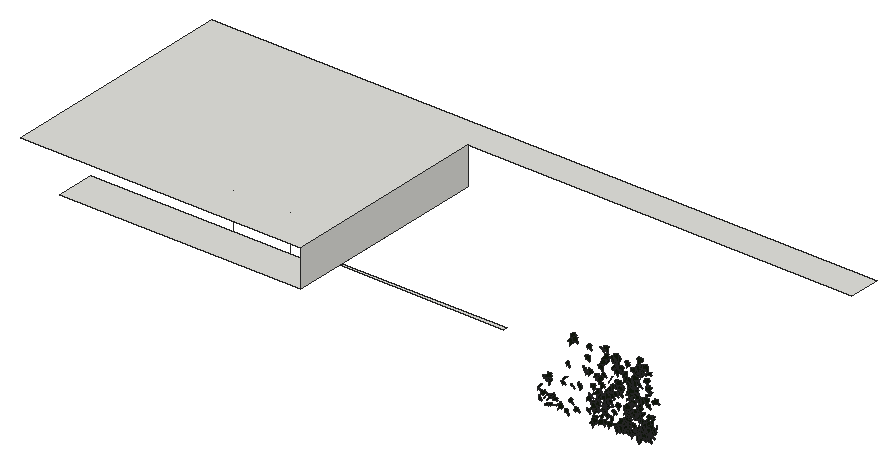
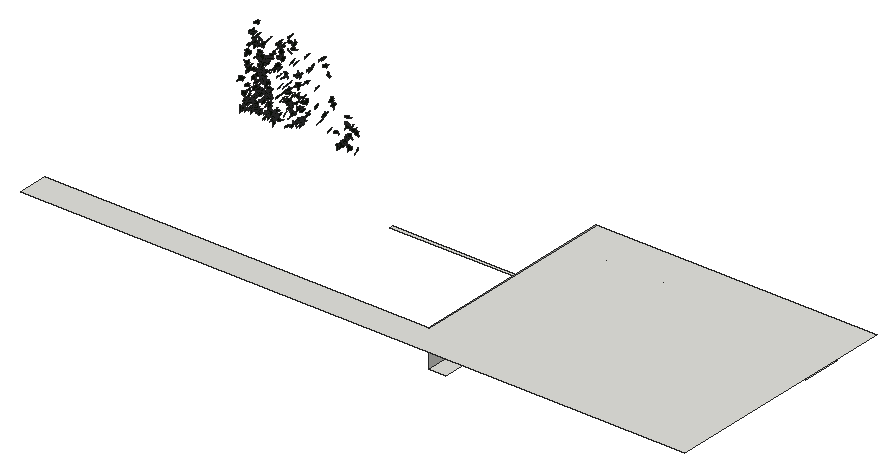
# SketchUp Ruby script. Lengths in inches.
U = 1.inch
M = Sketchup.active_model
def pt(a) = Geom::Point3d.new(a.map { |v| v * U })
def face(e, loops, mat)
  f = e.add_face(loops[0].map { |a| pt(a) })
  loops[1..].each { |l| e.add_face(l.map { |a| pt(a) }).erase! }
  f.material = f.back_material = mat if mat
  f
end
# faces: each face lists its corners as indices into pts; further lists are holes
def faces(e, pts, list, mat = nil) = list.each { |f| face(e, (f[0].is_a?(Array) ? f : [f]).map { |l| l.map { |i| pts[i] } }, mat) }
# xy, xz, yz: faces in a plane at the given z, y or x. An outline is a flat list of corners, or four numbers for a rectangle; further outlines are holes
def ring(l) = l.size == 4 ? [[l[0], l[1]], [l[2], l[1]], [l[2], l[3]], [l[0], l[3]]] : l.each_slice(2).to_a
def flat(e, list, mat, &to3) = list.each { |f| face(e, (f[0].is_a?(Array) ? f : [f]).map { |l| ring(l).map { |u, v| to3.(u, v) } }, mat) }
def xy(e, z, list, mat = nil) = flat(e, list, mat) { |x, y| [x, y, z] }
def xz(e, y, list, mat = nil) = flat(e, list, mat) { |x, z| [x, y, z] }
def yz(e, x, list, mat = nil) = flat(e, list, mat) { |y, z| [x, y, z] }
def lines(e, pts, list) = list.each { |a, b| e.add_line(pt(pts[a]), pt(pts[b])) }
# prism: a flat outline (further loops are holes) pulled along v
def prism(e, loops, v, mat = nil)
  f = face(e, loops, mat); d = Geom::Vector3d.new(v.map { |x| x * U })
  f.pushpull(f.normal.samedirection?(d) ? d.length : -d.length)
end
def box(e, o, s, mat = nil) = prism(e, [[o, [o[0] + s[0], o[1], o[2]], [o[0] + s[0], o[1] + s[1], o[2]], [o[0], o[1] + s[1], o[2]]]], [0, 0, s[2]], mat)
def at(x, y, z, deg = 0) = Geom::Transformation.translation(pt([x, y, z])) * Geom::Transformation.rotation(ORIGIN, Z_AXIS, deg.degrees)
def axes(o, x, y, z) = Geom::Transformation.new([*x, 0, *y, 0, *z, 0, *pt(o).to_a, 1])
def part(name) = M.definitions.add(name)
# library, detail: a bought-in or finely detailed component or shape, given as its bounding box
def library(name, o, s) = part(name).tap { |d| box(d.entities, o, s) }
def detail(e, o, s) = box(e.add_group.entities, o, s)
def put(e, d, t, mat = nil) = e.add_instance(d, t).tap { |i| i.material = mat if mat }
def group(e, t, mat = nil) = e.add_group.tap { |g| g.transformation = t; g.material = mat if mat }.entities
root = M.entities
M.materials.add("efeu1").color = [18, 25, 13]
c1 = part("ivyleaf_9")
p = [[1.54,2.16,1.25],[1.36,2.04,1.19],[-0.21,0.99,0.68],[-0.71,1.11,0.82],[-0.85,0.86,0.67],[-0.8,0.17,0.21],
  [-0.9,-0.01,0.1],[-0.67,-0.16,-0.02],[-0.08,-0.08,-0.05],[-0.03,-0.6,-0.4],[0.65,-0.88,-0.66],[0.83,-0.6,-0.49],
  [1.29,-0.42,-0.43],[1.8125,-0.07,-0.26],[1.21,0.44,0.15]]
faces(c1.entities,p,[[0,1,2,3,4,5,6,7,8,9,10,11,12,13,14]],"efeu1")
xy(root,328.1875,[[63.85,139.625,270.19,172.6875],[255.63,172.6875,270.19,181.4375],[270.19,181.4375,411.76,184.12],[255.63,184.12,270.19,319]])
xy(root,360,[[29.66,139.625,270.19,139.625,270.19,319,600,319,600,345.4375,29.66,345.4375]])
yz(root,270.19,[[139.625,328.1875,319,360]])
p = [[186.23,172.6875,360],[186.23,172.6875,328.1875],[235.22,172.6875,360],[235.22,172.6875,328.1875]]
lines(root,p,[[0,1],[2,3]])
put(root,c1,axes([491.06,119.55,331.81],[0.98321,-0.43675,-0.79022],[-0.6769,0.44134,-1.04482],[0.6616,1.10061,0.10539]))
put(root,c1,axes([494.23,116.77,342.93],[-0.50471,0.9603,-0.79093],[0.29874,-0.71022,-1.10944],[-1.2888,-0.54069,0.05257]))
put(root,c1,axes([494.78,120.51,348.57],[0.8379,-1.02369,-0.06234],[-0.00036,0.07491,-1.33503],[1.10748,0.77453,0.04673]))
put(root,c1,axes([499.15,117.69,329.99],[0.74075,1.01696,0.13512],[0.07482,0.10999,-1.2757],[-1.10472,0.68936,0.00421]))
put(root,c1,axes([499.41,119.17,347.66],[0.9407,0.95541,0.26934],[-0.05629,0.38876,-1.3092],[-1.06759,0.82135,0.30636]))
put(root,c1,axes([500.5,113.04,340.41],[0.17657,0.26151,1.32901],[-1.3928,0.22553,0.1236],[-0.21124,-1.26842,0.29598]))
put(root,c1,axes([500.88,120.67,335.94],[-0.15345,1.13375,-0.52577],[-0.03576,-0.51213,-1.18477],[-1.34019,-0.11615,0.09182]))
put(root,c1,axes([501.08,116.4375,338.25],[-0.68537,0.89054,-0.64163],[0.04243,-0.69561,-1.08628],[-1.16927,-0.54723,0.33667]))
put(root,c1,axes([500.22,119.6875,348.3],[-0.81391,-0.69586,-0.81701],[0.86609,0.24203,-1.02303],[0.73112,-1.06137,0.30237]))
put(root,c1,axes([501.71,121.67,334.63],[-0.43261,0.2825,1.18213],[-1.00858,0.648,-0.50976],[-0.76344,-1.01615,0.00357]))
put(root,c1,axes([500.99,119.21,348.96],[-1.09001,-0.37422,-0.73907],[0.73045,0.21948,-1.11918],[0.46779,-1.21469,0.02546]))
put(root,c1,axes([502.0625,118.14,352.8],[-1.15304,-0.11068,0.76991],[-0.75428,-0.31667,-1.09673],[0.29085,-1.26,0.20801]))
put(root,c1,axes([502.59,115.34,335.8],[0.51297,0.78721,0.95609],[0.19946,0.92887,-0.92644],[-1.29182,0.45601,0.23661]))
put(root,c1,axes([502.41,122.02,332.98],[0.89619,0.87408,0.14744],[0.1088,0.09984,-1.25343],[-0.95013,0.83588,-0.00446]))
put(root,c1,axes([504.23,114.77,332.87],[1.11009,0.20793,0.82745],[0.82025,0.24831,-1.08792],[-0.34055,1.27588,0.07688]))
put(root,c1,axes([506.18,121.38,330.43],[0.12532,1.05764,0.69606],[-0.04469,0.67503,-1.10193],[-1.35101,0.07578,0.10101]))
put(root,c1,axes([514.375,114.71,335.34],[-1.21116,-0.52096,0.19612],[-0.1902,-0.05406,-1.31821],[0.52315,-1.22574,-0.02521]))
put(root,c1,axes([517.23,112.87,355.13],[0.79088,0.38712,-1.07511],[-1.00802,-0.37942,-0.87815],[-0.53815,1.2796,0.06487]))
put(root,c1,axes([517.92,112.67,357.73],[0.58616,0.65304,1.08802],[0.47943,0.99569,-0.85591],[-1.1749,0.7321,0.19356]))
put(root,c1,axes([517.82,120.96,349.81],[1.09478,-0.78677,0.26516],[0.2539,-0.10053,-1.34658],[0.79047,1.12194,0.06528]))
put(root,c1,axes([519.67,112.89,334.43],[0.65078,-1.15916,-0.29844],[-0.0944,0.28894,-1.32809],[1.19324,0.65505,0.05769]))
put(root,c1,axes([520.5,118.41,385.79],[-0.91086,-1.13881,0.03125],[-0.02038,-0.02372,-1.45827],[1.13906,-0.91109,-0.0011]))
put(root,c1,axes([521.77,118.1,391.04],[0.04989,-1.401,-0.45119],[0.17121,0.45391,-1.3905],[1.46187,-0.00535,0.17825]))
put(root,c1,axes([523.41,117.5,389.22],[0.1852,-1.18685,-0.84705],[0.38674,0.86326,-1.125],[1.4059,-0.08112,0.42105]))
put(root,c1,axes([523.42,109.72,373.73],[-0.03799,-0.29316,-1.43905],[1.43722,0.2886,-0.09674],[0.302,-1.41032,0.27934]))
put(root,c1,axes([524.04,112.02,344.46],[0.76113,-1.06438,-0.49172],[-0.16172,0.48534,-1.30088],[1.16126,0.76522,0.14113]))
put(root,c1,axes([525.49,120.44,353.23],[0.724,-1.03353,0.55169],[0.2756,-0.48009,-1.26106],[1.13868,0.77334,-0.04555]))
put(root,c1,axes([527.59,113.15,338.16],[0.80232,-0.79111,-0.80628],[-0.19572,0.87665,-1.05491],[1.11249,0.72477,0.39589]))
put(root,c1,axes([532.34,121.27,344.83],[0.40368,-1.09674,-0.68829],[-0.07448,0.7001,-1.15924],[1.29269,0.38282,0.14815]))
put(root,c1,axes([533.79,118.08,378.62],[0.54183,-1.18623,-0.64307],[-0.12496,0.64589,-1.29672],[1.34353,0.53846,0.13873]))
put(root,c1,axes([533.74,110.12,359.84],[0.25984,-1.28174,0.64002],[0.22372,-0.60618,-1.3048],[1.41507,0.3312,0.08876]))
put(root,c1,axes([535.62,119.13,368.05],[-0.55222,-1.3096,0.07111],[-0.01992,-0.06877,-1.42124],[1.31138,-0.55252,0.00835]))
put(root,c1,axes([535.74,117.19,387.75],[0.61048,-1.22558,-0.56432],[-0.00111,0.61894,-1.3454],[1.34926,0.55503,0.25422]))
put(root,c1,axes([535.8,121.87,337.8125],[0.39608,-0.95937,0.84674],[0.3218,-0.78321,-1.03792],[1.23847,0.51033,-0.00111]))
put(root,c1,axes([537.04,120.18,356.61],[0.00922,-1.33902,-0.38342],[0.01688,0.38351,-1.33892],[1.39273,0.00421,0.01877]))
put(root,c1,axes([536.73,116.47,351.33],[1.29715,-0.55053,0.23449],[0.21062,-0.1039,-1.40908],[0.56009,1.31407,-0.01317]))
put(root,c1,axes([537.36,109.94,375.16],[1.0725,-1.04548,-0.03075],[-0.0239,0.01953,-1.49776],[1.04566,1.07276,-0.0027]))
put(root,c1,axes([537.8125,114.01,340.61],[0.57296,-1.14178,0.59781],[0.41423,-0.45636,-1.26865],[1.22043,0.69093,0.14994]))
put(root,c1,axes([539.49,121.83,339.83],[-1.34684,-0.00456,0.09388],[-0.09385,-0.00694,-1.34683],[0.00503,-1.35009,0.00661]))
put(root,c1,axes([538.35,111.18,371.94],[0.12554,-1.21301,0.85578],[0.26277,-0.82712,-1.21092],[1.46106,0.25298,0.14425]))
put(root,c1,axes([539.84,121.57,338.15],[-0.73475,-1.00394,0.51386],[-0.30506,-0.41352,-1.24409],[1.08577,-0.79557,-0.00181]))
put(root,c1,axes([539.1,121.5625,339.9],[0.3193,-1.07225,-0.76696],[0.15763,0.81452,-1.07313],[1.30886,0.16349,0.31634]))
put(root,c1,axes([539.65,118.93,344.67],[-0.49458,-1.26783,0.04544],[-0.00699,-0.04605,-1.36085],[1.26863,-0.49452,0.01022]))
put(root,c1,axes([539.65,119.3,333.49],[-0.08067,-1.21087,-0.54346],[0.20773,0.52624,-1.20332],[1.31088,-0.15791,0.15725]))
put(root,c1,axes([540.33,120.63,346.7],[0.42987,-0.73139,-1.07949],[-0.23869,1.0733,-0.82225],[1.2819,0.44511,0.20889]))
put(root,c1,axes([542.24,119.26,364.2],[0.06702,1.41664,-0.05834],[-0.00082,-0.05837,-1.41823],[-1.41784,0.067,-0.00194]))
put(root,c1,axes([543.33,118.47,344.83],[-0.73484,-0.28673,1.11502],[-0.96495,-0.56812,-0.78203],[0.62797,-1.20851,0.10308]))
put(root,c1,axes([542.84,113.71,333.02],[-0.56445,-1.32849,-0.20518],[0.09095,0.18428,-1.44338],[1.34116,-0.57162,0.01152]))
put(root,c1,axes([542.84,120.52,350.21],[-0.26979,-1.3436,-0.18841],[0.01274,0.18958,-1.3702],[1.35668,-0.26897,-0.0246]))
put(root,c1,axes([544.11,121.46,334.64],[-0.76329,0.95569,0.57248],[-0.37002,0.43708,-1.223],[-1.05079,-0.84812,0.01482]))
put(root,c1,axes([543.71,113.74,335.36],[-0.46046,-1.26984,-0.02353],[-0.0079,0.02789,-1.35064],[1.27003,-0.46022,-0.01693]))
put(root,c1,axes([544.38,112.42,346.89],[-1.06212,-0.92998,0.44622],[-0.30903,-0.32417,-1.4112],[0.98411,-1.1055,0.03845]))
put(root,c1,axes([544.59,118.63,354.44],[-1.30914,-0.45963,-0.17804],[0.16026,0.08089,-1.38729],[0.46612,-1.31872,-0.02305]))
put(root,c1,axes([544.26,115.54,369.02],[-0.09958,-1.46951,-0.22114],[0.12992,0.21218,-1.46846],[1.48037,-0.11747,0.114]))
put(root,c1,axes([544.1875,114.82,366.9],[-0.19262,0.41185,1.41968],[0.62963,-1.27246,0.45457],[1.33742,0.65837,-0.00954]))
put(root,c1,axes([545.0625,116.96,353.93],[-0.21059,-1.3596,0.21791],[-0.06245,-0.21078,-1.3755],[1.37553,-0.21772,-0.02909]))
put(root,c1,axes([546.36,120.9,342.64],[-1.35822,-0.18615,0.01166],[-0.00507,-0.04877,-1.37009],[0.18644,-1.35739,0.04763]))
put(root,c1,axes([545.75,116.85,333],[0.23775,-0.63453,-1.24816],[-0.0975,1.25544,-0.65681],[1.39679,0.19564,0.1666]))
put(root,c1,axes([546.14,119.17,360.43],[-0.48389,-1.23962,0.49954],[-0.01822,-0.5251,-1.32071],[1.33636,-0.45602,0.16287]))
put(root,c1,axes([546.32,120.65,331.78],[-0.02987,-1.31064,-0.22703],[0.04879,0.22586,-1.31027],[1.32926,-0.03774,0.04299]))
put(root,c1,axes([546.4,120.81,341.39],[-0.79827,-0.58379,-0.95076],[0.7634,0.56673,-0.98896],[0.81362,-1.10454,-0.00491]))
put(root,c1,axes([546.9,115.72,368.06],[-0.76626,-1.26593,-0.27277],[0.13242,0.23868,-1.47974],[1.28819,-0.77756,-0.01014]))
put(root,c1,axes([547.66,120.25,346.92],[-0.43565,1.30172,0.21151],[-0.07545,0.19778,-1.37266],[-1.31663,-0.44205,0.00868]))
put(root,c1,axes([546.97,120.5,345.48],[0.41961,-1.30874,0.10938],[0.02131,-0.10802,-1.37431],[1.31313,0.41996,-0.01265]))
put(root,c1,axes([547.01,115.55,377.09],[0.44048,-1.33393,-0.39082],[0.04365,0.42305,-1.39473],[1.38932,0.40963,0.16773]))
put(root,c1,axes([548.52,112.09,359.16],[-1.14594,-0.38162,0.74556],[-0.65746,-0.37291,-1.2014],[0.51889,-1.31529,0.1243]))
put(root,c1,axes([547.4,121.18,337.97],[0.40046,-1.2942,-0.11492],[0.07446,0.14291,-1.35003],[1.29716,0.39135,0.11297]))
put(root,c1,axes([547.74,120.38,347.16],[0.1495,-1.3587,-0.23646],[-0.00123,0.23772,-1.36669],[1.37913,0.1475,0.02441]))
put(root,c1,axes([548.58,120.67,344.11],[-0.53144,-1.22449,-0.33365],[0.10004,0.32018,-1.3344],[1.26519,-0.53966,-0.03464]))
put(root,c1,axes([548.23,117.41,352.58],[0.49896,-1.29655,-0.07612],[-0.01852,0.07443,-1.38921],[1.29865,0.49921,0.00943]))
put(root,c1,axes([548.57,115.51,390.3],[1.28415,-0.54338,-0.53235],[0.49245,-0.20228,1.39438],[-0.57979,-1.37533,0.00525]))
put(root,c1,axes([549.17,120.35,347.43],[-0.18004,-1.37168,0.08],[0.00557,-0.08141,-1.38335],[1.374,-0.1794,0.01609]))
put(root,c1,axes([549.84,122.29,330.59],[-0.41488,-1.24005,0.23911],[0.02109,-0.25846,-1.30375],[1.26272,-0.40311,0.10034]))
put(root,c1,axes([549.92,119.85,355.05],[-0.66417,-1.19263,-0.35048],[0.29432,0.23519,-1.35808],[1.20772,-0.71319,0.13823]))
put(root,c1,axes([550.86,119.23,357.02],[-0.45888,-1.3419,0.0499],[0.00555,-0.05463,-1.41801],[1.34282,-0.45834,0.02291]))
put(root,c1,axes([551.22,117.83,346.42],[0.92221,-0.22884,1.07308],[1.08452,-0.02249,-0.93683],[0.16641,1.41473,0.15868]))
put(root,c1,axes([551.92,119.37,355.77],[0.22405,-1.38648,-0.15003],[0.01643,0.15456,-1.40388],[1.39448,0.22094,0.04064]))
put(root,c1,axes([551.95,120.04,350.02],[0.73144,-1.16552,-0.24444],[-0.00873,0.28161,-1.36887],[1.19085,0.71794,0.14011]))
put(root,c1,axes([553.52,111.91,384.13],[-1.31169,-0.42145,0.57101],[-0.40666,-0.53709,-1.33056],[0.58164,-1.32595,0.35746]))
put(root,c1,axes([552.33,119.125,359.71],[0.7425,-1.04326,-0.62084],[-0.05781,0.69654,-1.2396],[1.21264,0.67199,0.32104]))
put(root,c1,axes([554.07,113.72,382.65],[0.07518,0.77287,1.25945],[-0.69178,1.13276,-0.65383],[-1.30576,-0.55563,0.41891]))
put(root,c1,axes([553.06,110.86,374.84],[1.10105,-0.55116,-0.78981],[-0.50791,0.68695,-1.18744],[0.81829,1.16799,0.32569]))
put(root,c1,axes([554.18,117.99,368.17],[-0.77945,1.18919,-0.29571],[0.1738,-0.23963,-1.4218],[-1.21302,-0.79847,-0.0137]))
put(root,c1,axes([553.37,119.94,337.17],[0.11202,-1.0973,0.79828],[0.07097,-0.79516,-1.10297],[1.35509,0.13236,-0.00822]))
put(root,c1,axes([553.45,119.66,354.84],[0.7894,-1.09313,-0.41091],[-0.01398,0.4871,-1.32267],[1.16773,0.7448,0.26195]))
put(root,c1,axes([553.58,113.3,394.86],[0.32174,-1.42081,-0.39279],[0.04557,0.41144,-1.45091],[1.4734,0.29753,0.13065]))
put(root,c1,axes([554.42,113.71,350.64],[-0.17262,0.80836,1.24038],[0.02741,-1.24682,0.81637],[1.48028,0.11735,0.12953]))
put(root,c1,axes([556.02,111.97,388.9],[-1.45196,-0.00649,0.40098],[-0.401,0.04278,-1.45134],[-0.00514,-1.50571,-0.04296]))
put(root,c1,axes([554.9375,113.98,357.45],[-0.41628,-1.1614,0.84505],[-0.07715,-0.86048,-1.22061],[1.43423,-0.38338,0.17962]))
put(root,c1,axes([556.46,118.52,363.5],[-0.65955,-1.19456,0.45534],[0.00417,-0.51437,-1.3434],[1.27839,-0.61462,0.2393]))
put(root,c1,axes([557.92,121.16,332.03],[-0.68805,0.31455,1.08157],[-1.12576,-0.23406,-0.6481],[0.03734,-1.26033,0.3903]))
put(root,c1,axes([556.49,117.54,377.43],[0.34207,0.23819,1.41732],[0.99117,1.01591,-0.40995],[-1.04073,1.04582,0.07542]))
put(root,c1,axes([557.01,118.91,357.79],[0.85726,-1.00618,-0.51554],[-0.13791,0.54909,-1.30099],[1.12213,0.83617,0.23396]))
put(root,c1,axes([558.49,116.65,383.05],[1.12006,0.3491,-0.93058],[-0.9448,-0.0613,-1.16017],[-0.30856,1.45491,0.17441]))
put(root,c1,axes([557.97,115.76,387.14],[0.06298,-1.46571,0.35331],[0.074,-0.35019,-1.46594],[1.50587,0.07851,0.05726]))
put(root,c1,axes([558.52,116.68,344.98],[-0.12969,-1.22769,0.81297],[0.24358,-0.82276,-1.20362],[1.45217,0.02836,0.27449]))
put(root,c1,axes([558.95,120.05,349.25],[0.09886,-1.39101,0.07323],[-0.00058,-0.07346,-1.3945],[1.39293,0.09869,-0.00577]))
put(root,c1,axes([559.33,116.27,386.41],[-0.56031,-1.24057,-0.64669],[0.24405,0.59927,-1.36106],[1.37756,-0.61076,-0.02191]))
put(root,c1,axes([559.3,118.25,364.26],[0.4243,-1.3398,-0.3065],[0.07468,0.34277,-1.39498],[1.37238,0.39557,0.17067]))
put(root,c1,axes([560.95,121.45,336.31],[-1.3038,0.23628,0.28342],[-0.2884,-0.00331,-1.32396],[-0.23017,-1.33425,0.05348]))
put(root,c1,axes([559.65,117.4,368.67],[0.62464,-1.28792,-0.23648],[-0.0168,0.2541,-1.42828],[1.30934,0.61768,0.09449]))
put(root,c1,axes([560.56,122.1,330.36],[0.21907,-0.20191,-1.28994],[-0.94684,0.87605,-0.29792],[0.89901,0.97185,0.00056]))
put(root,c1,axes([560.58,117.03,378.53],[-0.80645,-1.2066,0.28178],[0.09614,-0.39612,-1.42109],[1.23533,-0.75687,0.29455]))
put(root,c1,axes([560.21,115.95,389.48],[0.19445,-1.48559,-0.22501],[0.12493,0.24209,-1.49037],[1.49733,0.17273,0.15357]))
put(root,c1,axes([560.66,117.4,333.17],[-0.34578,-1.39142,0.23096],[-0.02294,-0.23222,-1.43336],[1.41028,-0.34493,0.03331]))
put(root,c1,axes([562.08,121.59,334.72],[-1.33461,0.10417,-0.0331],[0.02478,-0.10659,-1.3346],[-0.10646,-1.33076,0.1043]))
put(root,c1,axes([561.22,120.38,331.32],[-0.13897,-1.01556,-0.92303],[0.1021,0.91753,-1.02487],[1.36855,-0.17158,-0.01727]))
put(root,c1,axes([561.3,115.62,378.08],[0.24661,-1.45658,0.09217],[0.00293,-0.09299,-1.47725],[1.45949,0.2463,-0.01261]))
put(root,c1,axes([561.31,121.625,332.23],[1.31464,0.01191,0.05278],[0.05258,0.02135,-1.31453],[-0.01276,1.31553,0.02085]))
put(root,c1,axes([561.59,116.03,387.56],[-0.32029,-1.40382,-0.44375],[0.12811,0.42583,-1.4396],[1.4667,-0.34376,0.02884]))
put(root,c1,axes([561.77,122.18,332.33],[-0.29071,-1.29724,-0.0253],[0.01382,0.02283,-1.32939],[1.29742,-0.29092,0.00849]))
put(root,c1,axes([563.03,121.72,336.55],[0.48247,1.23788,0.21388],[0.01185,0.22461,-1.32676],[-1.25617,0.47757,0.06963]))
put(root,c1,axes([562.84,114.78,370.02],[0.17714,-0.46759,-1.38586],[0.07074,1.39709,-0.46234],[1.46091,-0.01095,0.19043]))
put(root,c1,axes([563.58,116.46,335.37],[-0.63544,-1.12986,-0.38183],[0.31356,0.25915,-1.28867],[1.15068,-0.69456,0.14031]))
put(root,c1,axes([563.92,121.88,335.88],[-0.15442,-1.31308,-0.17275],[0.07784,0.16462,-1.32087],[1.3221,-0.16306,0.05759]))
put(root,c1,axes([564.01,116.6,381.31],[0.30832,-1.44235,-0.23538],[0.01161,0.24297,-1.47366],[1.46138,0.30237,0.06137]))
put(root,c1,axes([564.33,116.51,335.16],[0.05159,-1.35301,0.57577],[0.05556,-0.57392,-1.35364],[1.46937,0.0692,0.03097]))
put(root,c1,axes([564.2,121.47,338.92],[0.715,-1.12468,0.2344],[0.17075,-0.16899,-1.33168],[1.13609,0.73322,0.05263]))
put(root,c1,axes([565.39,121.15,342.1],[0.20658,1.23635,0.53611],[-0.04626,0.54856,-1.24723],[-1.34679,0.1708,0.12507]))
put(root,c1,axes([565.24,118.66,334.5],[0.61803,1.20184,0.31688],[0.13007,0.28941,-1.35134],[-1.23609,0.63136,0.01624]))
put(root,c1,axes([565.28,116.08,366.45],[-0.27546,-1.3882,-0.32804],[0.04447,0.32559,-1.41513],[1.42574,-0.27836,-0.01924]))
put(root,c1,axes([565.12,120.93,331.96],[0.36284,-1.20489,-0.44179],[-0.03576,0.44944,-1.25512],[1.28284,0.35332,0.08997]))
put(root,c1,axes([565.3,114.52,367.01],[0.0349,-1.49386,0.11893],[0.0183,-0.11853,-1.49419],[1.49848,0.03624,0.01548]))
put(root,c1,axes([565.45,119.73,340.38],[0.16823,-1.32871,0.17319],[-0.00564,-0.17525,-1.33904],[1.33994,0.16609,-0.02738]))
put(root,c1,axes([565.98,122.24,337.09],[-0.73809,-1.01334,0.44205],[0.02337,-0.5457,-1.2119],[1.10531,-0.66513,0.32081]))
put(root,c1,axes([566.89,120.375,346.65],[-1.27494,-0.41448,0.3082],[-0.28945,-0.10647,-1.34057],[0.42778,-1.30733,0.01146]))
put(root,c1,axes([565.95,119,350.48],[0.33043,-1.30908,-0.36857],[-0.08169,0.3595,-1.35011],[1.35752,0.34027,0.00846]))
put(root,c1,axes([565.92,119.04,345.95],[0.89229,0.56573,0.94393],[0.71826,0.62131,-1.05134],[-0.83376,1.14068,0.1045]))
put(root,c1,axes([566.88,119.72,348.84],[-1.00858,0.60212,-0.72264],[0.57707,-0.4406,-1.17253],[-0.74279,-1.15987,0.07027]))
put(root,c1,axes([566.67,116.89,377.72],[-0.5201,-1.35354,-0.31276],[0.07362,0.30663,-1.44946],[1.38725,-0.52373,-0.04033]))
put(root,c1,axes([566.42,112.6,364.98],[0.44061,-1.25473,-0.59867],[-0.17299,0.57366,-1.32962],[1.37943,0.47272,0.02448]))
put(root,c1,axes([566.68,118.47,340.09],[-0.31422,0.76039,1.16127],[0.08835,-1.17728,0.79478],[1.38525,0.24757,0.21272]))
put(root,c1,axes([566.6,121.66,336.33],[-0.029,-1.31423,-0.28767],[0.05064,0.28647,-1.31383],[1.34439,-0.03914,0.04329]))
put(root,c1,axes([566.89,120.12,347.125],[0.08993,-1.21194,-0.83529],[0.02267,0.83789,-1.21327],[1.47173,0.06115,0.06973]))
put(root,c1,axes([568.52,119.06,351.88],[-1.22294,-0.57852,0.32969],[-0.30178,-0.13302,-1.35284],[0.59355,-1.25959,-0.00855]))
put(root,c1,axes([567.92,119.4,356.97],[0.93933,1.02694,0.18715],[0.10397,0.15848,-1.39142],[-1.03866,0.94459,0.02998]))
put(root,c1,axes([567.6,120.01,332.72],[-0.00774,-1.08691,-0.78547],[0.5153,0.72277,-1.00522],[1.23807,-0.30761,0.41348]))
put(root,c1,axes([567.86,120.77,349.62],[0.5191,-1.22683,-0.33742],[0.09416,0.40046,-1.31118],[1.2689,0.47218,0.23533]))
put(root,c1,axes([568.13,120.39,349.12],[-0.70299,-0.31713,-1.14848],[1.02871,0.5112,-0.77084],[0.6011,-1.24574,-0.02396]))
put(root,c1,axes([569.1,117.32,373.89],[-1.15365,-0.7999,0.43441],[-0.10709,-0.57717,-1.34716],[0.90392,-1.08926,0.39482]))
put(root,c1,axes([569.125,121.82,330],[0.01163,-1.31954,-0.03233],[0.00646,0.03239,-1.31957],[1.31992,0.01147,0.00674]))
put(root,c1,axes([570.07,119.73,358.22],[-1.33698,0.42942,-0.05658],[-0.05187,0.02352,1.40424],[0.43002,1.33797,-0.00652]))
put(root,c1,axes([569.37,120.51,345.47],[-0.24259,-1.32443,0.16967],[-0.01885,-0.16903,-1.34642],[1.33512,-0.24304,0.01182]))
put(root,c1,axes([569.09,119.07,339.24],[0.68133,-1.17117,-0.11113],[-0.04584,0.10189,-1.35489],[1.17554,0.68277,0.01157]))
put(root,c1,axes([569.625,121.22,345.67],[0.83182,-1.04884,-0.25108],[0.03173,0.34075,-1.3183],[1.07801,0.79929,0.23255]))
put(root,c1,axes([569.81,117.6875,363.64],[0.09755,-1.36693,-0.36073],[0.13283,0.36885,-1.36178],[1.40747,0.05993,0.15352]))
put(root,c1,axes([570.21,118.23,370.1],[-0.41873,-1.34091,0.34966],[0.0156,-0.36981,-1.39951],[1.38566,-0.40104,0.12142]))
put(root,c1,axes([569.96,119.11,333.26],[0.25643,-1.17328,-0.65489],[0.11505,0.68343,-1.17937],[1.33874,0.166,0.22679]))
put(root,c1,axes([570.38,115.78,387.29],[-0.18882,-1.3491,0.65494],[0.09642,-0.66966,-1.35163],[1.49656,-0.12707,0.16971]))
put(root,c1,axes([570.44,116.21,342.51],[-0.47407,-0.12342,1.36757],[1.37017,0.05229,0.47969],[-0.08998,1.44646,0.09935]))
put(root,c1,axes([572.24,117.33,363.31],[-1.21754,0.26805,0.70615],[-0.72336,-0.02834,-1.23646],[-0.21735,-1.40721,0.15941]))
put(root,c1,axes([570.75,119.73,355.86],[0.06066,-1.40388,-0.04886],[-0.00004,0.04891,-1.40519],[1.40473,0.06062,0.00207]))
put(root,c1,axes([570.6875,117.25,373.85],[0.26298,-1.4373,-0.12505],[-0.01504,0.12437,-1.46114],[1.44265,0.26331,0.00756]))
put(root,c1,axes([571.5,119.3,359.85],[0.51963,1.27378,0.34985],[0.01436,0.37048,-1.37021],[-1.32087,0.50513,0.12274]))
put(root,c1,axes([572.07,119.49,358.7],[-0.1231,1.38655,0.24644],[-0.01839,0.24578,-1.392],[-1.40816,-0.12442,-0.00337]))
put(root,c1,axes([570.85,114.95,346.61],[1.0029,-0.63853,0.94186],[0.77488,-0.53615,-1.18858],[0.83329,1.26706,-0.0283]))
put(root,c1,axes([572.58,118.1,369.56],[0.82794,1.16374,0.19694],[0.10514,0.16689,-1.42817],[-1.17559,0.83452,0.01097]))
put(root,c1,axes([573.01,122.38,334.3],[-0.11273,-1.27477,0.33346],[0.04378,-0.33811,-1.27777],[1.31694,-0.09788,0.07102]))
put(root,c1,axes([573.98,118.13,374.56],[-0.11581,1.44759,-0.09005],[0.01959,-0.08877,-1.45216],[-1.45026,-0.1168,-0.01242]))
put(root,c1,axes([573.67,118.12,357.87],[-0.58248,-1.25982,-0.26242],[0.30596,0.14421,-1.37146],[1.24996,-0.62238,0.21341]))
put(root,c1,axes([573.59,118.43,348.52],[-0.00343,-1.39002,0.04837],[-0.00357,-0.04836,-1.39002],[1.39085,-0.00355,-0.00345]))
put(root,c1,axes([574.35,118.68,365.8],[0.33664,1.3601,-0.31395],[-0.0449,-0.31223,-1.4008],[-1.39514,0.33823,-0.03067]))
put(root,c1,axes([575.39,115.7,370.55],[-1.21057,0.18215,0.78668],[-0.8029,-0.12042,-1.20764],[-0.08607,-1.4387,0.20068]))
put(root,c1,axes([574.27,119.32,362.77],[-0.67062,-1.19066,0.37379],[0.00724,-0.42805,-1.3505],[1.24793,-0.63736,0.20871]))
put(root,c1,axes([573.98,116.98,383.48],[0.05956,-1.41374,-0.45576],[-0.00751,0.45584,-1.41495],[1.48537,0.059,0.01112]))
put(root,c1,axes([574.28,117.37,340.42],[0.28628,-1.37135,0.00656],[-0.01647,-0.01014,-1.40079],[1.37126,0.28617,-0.01819]))
put(root,c1,axes([573.97,117.46,356.33],[0.98273,-0.96991,0.26855],[0.39691,0.02861,-1.34916],[0.92482,1.01836,0.29367]))
put(root,c1,axes([574.52,117.53,366.3125],[0.74911,-0.92857,-0.8013],[-0.3484,0.73916,-1.18227],[1.17599,0.81049,0.16017]))
put(root,c1,axes([575.77,119.43,333.98],[-1.27213,0.60102,-0.08894],[0.07574,-0.0479,-1.40691],[-0.60282,-1.27433,0.01093]))
put(root,c1,axes([575.53,118.55,367.54],[-0.40209,1.00373,-0.95074],[0.22909,-0.92808,-1.07669],[-1.36342,-0.45195,0.09948]))
put(root,c1,axes([574.95,117.25,372.41],[-0.43461,-1.39965,0.00399],[0.02439,-0.01175,-1.46533],[1.39944,-0.43447,0.02677]))
put(root,c1,axes([575.22,121.53,331.61],[-0.98476,-0.84722,-0.36204],[0.35238,0.14329,-1.29379],[0.85129,-1.03937,0.11674]))
put(root,c1,axes([574.9375,118.44,344.38],[0.31695,-0.26386,1.3366],[1.33972,0.30972,-0.25654],[-0.24756,1.3383,0.3229]))
put(root,c1,axes([575.67,117.77,373.26],[-0.37242,-1.41411,0.01021],[0.01607,-0.01479,-1.4622],[1.41406,-0.37227,0.0193]))
put(root,c1,axes([576.73,118.11,371.78],[-0.46116,1.34459,0.30251],[-0.05205,0.30178,-1.42068],[-1.37721,-0.46165,-0.0476]))
put(root,c1,axes([577.01,116.75,376.18],[-0.18313,1.39929,0.38168],[-0.35076,0.33057,-1.38019],[-1.40736,-0.26446,0.29432]))
put(root,c1,axes([577.32,118.25,373.74],[-0.92413,1.11126,0.13863],[-0.2163,-0.00076,-1.43574],[-1.09879,-0.93447,0.16603]))
put(root,c1,axes([575.66,118.14,367.6],[0.72579,-1.2362,-0.16537],[0.12303,0.26136,-1.41381],[1.24113,0.697,0.23685]))
put(root,c1,axes([576.87,112.02,370.08],[-1.21337,-0.79616,0.1212],[-0.10215,-0.06525,-1.45125],[0.79882,-1.21766,-0.00148]))
put(root,c1,axes([576.4375,119.98,349],[-0.57519,-1.23427,0.15405],[-0.04141,-0.15062,-1.36147],[1.24316,-0.5761,0.02592]))
put(root,c1,axes([576.38,120.05,344.79],[0.32747,-1.30622,0.20665],[0.04323,-0.2022,-1.34663],[1.32176,0.33023,-0.00716]))
put(root,c1,axes([575.78,113.83,336.8],[0.86217,-0.2815,1.21489],[1.19996,-0.21485,-0.90136],[0.33952,1.47415,0.10062]))
put(root,c1,axes([577.51,120.43,334.52],[-0.74735,-1.12046,-0.07532],[0.03576,0.06669,-1.34682],[1.12242,-0.74817,-0.00724]))
put(root,c1,axes([577.63,120.22,337.8125],[-0.53667,-1.23264,-0.08332],[0.02253,0.08107,-1.34435],[1.23525,-0.53701,-0.01169]))
put(root,c1,axes([577.62,119.83,353.76],[-0.28101,-1.36172,-0.12119],[0.00835,0.12202,-1.39032],[1.36708,-0.28065,-0.01642]))
put(root,c1,axes([577.92,116.69,380.42],[-0.82578,-1.21139,0.28154],[0.03038,-0.3575,-1.44911],[1.2433,-0.79585,0.22241]))
put(root,c1,axes([577.54,121.24,343.31],[0.22944,-1.32212,-0.17693],[-0.0039,0.17887,-1.34162],[1.3339,0.22793,0.02651]))
put(root,c1,axes([578.32,114.375,379.78],[-1.2666,-0.76159,-0.10938],[0.11756,0.01663,-1.47722],[0.76037,-1.27121,0.0462]))
put(root,c1,axes([577.68,116.61,350.37],[-0.25216,-1.15811,0.72503],[0.21254,-0.76155,-1.14252],[1.34971,-0.09644,0.31536]))
put(root,c1,axes([577.91,119.1875,333.95],[1.18329,0.61737,0.26006],[0.23236,0.11684,-1.33465],[-0.62832,1.20588,-0.00382]))
put(root,c1,axes([577.92,117.59,373.18],[1.05026,-0.95702,-0.27557],[0.02795,0.42865,-1.38215],[0.99551,0.99761,0.32952]))
put(root,c1,axes([579.85,114.88,384.97],[-1.46943,0.20864,-0.05049],[0.0523,0.00914,-1.48408],[-0.20819,-1.47027,-0.01639]))
put(root,c1,axes([579.34,120.07,348.91],[0.00163,-0.55664,-1.39819],[0.56866,-1.2943,0.51594],[-1.39334,-0.52889,0.20893]))
put(root,c1,axes([579.05,118.125,361.79],[-0.37247,-1.29911,0.39715],[0.12547,-0.44295,-1.33124],[1.35265,-0.31664,0.23285]))
put(root,c1,axes([579.1,115.11,365.2],[-0.37042,-1.23949,0.69554],[0.10397,-0.74047,-1.2642],[1.4175,-0.26959,0.27448]))
put(root,c1,axes([578.6875,117.36,382.19],[0.44524,-1.24767,0.64284],[0.37502,-0.54414,-1.31584],[1.35251,0.5616,0.15324]))
put(root,c1,axes([580.08,116.77,357.72],[-0.41827,0.49888,-1.28167],[0.6966,-1.07824,-0.64703],[-1.18588,-0.80934,0.07198]))
put(root,c1,axes([580.08,116.82,381.96],[1.19067,0.73727,-0.42845],[-0.40657,-0.15599,-1.39828],[-0.74956,1.25576,0.07786]))
put(root,c1,axes([580.08,115.57,387.3],[-0.28681,-1.41103,0.41049],[0.04429,-0.42634,-1.43459],[1.46886,-0.26266,0.12341]))
put(root,c1,axes([580.47,124.5,378.35],[1.00913,1.07367,0.32391],[0.15452,0.29848,-1.47074],[-1.11077,1.01695,0.08968]))
put(root,c1,axes([580.55,120.51,334.22],[-0.0517,-1.35294,-0.0195],[0.00109,0.01948,-1.35393],[1.35308,-0.05171,0.00034]))
put(root,c1,axes([580.4375,122.375,333.32],[0.32947,-1.24322,-0.31249],[0.00929,0.32496,-1.28301],[1.28186,0.31718,0.08962]))
put(root,c1,axes([580.52,111.31,356],[0.67074,-1.24246,-0.16385],[-0.05084,0.15872,-1.41162],[1.25218,0.67198,0.03046]))
put(root,c1,axes([580.59,122.15,334.3125],[0.56794,-1.17667,-0.19996],[-0.0422,0.20151,-1.30565],[1.1928,0.56739,0.04901]))
put(root,c1,axes([581.09,118.84,331.48],[1.13463,0.88787,-0.20203],[-0.16303,-0.11948,-1.44072],[-0.89585,1.14627,0.00631]))
put(root,c1,axes([580.71,117.47,337.91],[0.17055,-1.19124,0.68306],[0.19912,-0.65957,-1.20001],[1.35867,0.2462,0.09013]))
put(root,c1,axes([581.22,117.57,340.72],[1.04642,-0.50201,-0.87336],[-0.72041,0.50729,-1.15475],[0.70413,1.26507,0.11648]))
put(root,c1,axes([580.85,117,382.98],[1.48316,0.07544,0.00278],[-0.01152,0.28027,-1.45835],[-0.0746,1.45645,0.28049]))
put(root,c1,axes([581.14,114.01,350.44],[0.28698,-1.30151,-0.45817],[0.10948,0.48798,-1.31761],[1.37545,0.23272,0.20047]))
put(root,c1,axes([581.4,116.26,383.83],[0.05337,-1.43775,0.38232],[-0.00389,-0.3827,-1.43863],[1.4877,0.05058,-0.01747]))
put(root,c1,axes([582.47,114.72,334.13],[-0.86307,1.00778,-0.3785],[0.22164,-0.30838,-1.32648],[-1.05345,-0.89054,0.03101]))
put(root,c1,axes([582.75,124.29,337.09],[-0.71488,-0.48135,1.08489],[-0.77165,-0.77378,-0.85179],[0.90179,-1.04369,0.13116]))
put(root,c1,axes([581.89,121.69,339.71],[-0.11561,-1.28429,0.3593],[-0.03205,-0.35786,-1.28948],[1.33322,-0.11997,0.00015]))
put(root,c1,axes([582.16,118.6,361.82],[-0.68028,-1.24426,0.0029],[-0.01322,0.00392,-1.41803],[1.2442,-0.68028,-0.01348]))
put(root,c1,axes([581.85,116.92,385.5],[-0.41767,-1.4134,0.1654],[0.25117,-0.24289,-1.44133],[1.4007,-0.3779,0.30777]))
put(root,c1,axes([583.22,119.28,336.76],[-1.29205,0.33889,0.37968],[-0.3674,0.09577,-1.33576],[-0.35216,-1.34327,0.00055]))
put(root,c1,axes([581.75,122.24,362.99],[0.69476,1.30743,-0.25893],[0.11701,0.23104,1.48055],[1.32768,-0.70452,0.00501]))
put(root,c1,axes([583.72,113.43,332.9],[-0.70129,1.08423,0.7221],[-0.50964,0.52637,-1.2853],[-1.19885,-0.858,0.12399]))
put(root,c1,axes([582.93,121.49,332.83],[-0.68843,-0.9011,0.6956],[-0.0871,-0.76883,-1.08217],[1.13502,-0.60555,0.33886]))
put(root,c1,axes([582.98,113.6875,395.56],[-0.70943,-1.32986,0.06257],[-0.03388,-0.05284,-1.50725],[1.3309,-0.71023,-0.00502]))
put(root,c1,axes([583.47,125.42,346.46],[0.75029,0.8819,-0.78644],[-0.61416,-0.50482,-1.15201],[-1.00948,0.96259,0.11636]))
put(root,c1,axes([584.625,124.92,342.75],[-0.8965,0.8789,0.58269],[-0.5269,0.28914,-1.24679],[-0.91344,-1.02938,0.1473]))
put(root,c1,axes([583.37,116.44,388.64],[-0.37139,-1.42641,-0.28886],[0.02562,0.29167,-1.47319],[1.45514,-0.36919,-0.04779]))
put(root,c1,axes([584.4,128.85,336.19],[0.21964,-0.11241,-1.4939],[-1.41256,0.48741,-0.24436],[0.49904,1.42913,-0.03417]))
put(root,c1,axes([583.79,116.67,388.65],[-0.99414,-1.10921,0.08797],[0.12206,-0.22597,-1.46984],[1.10598,-0.97211,0.24129]))
put(root,c1,axes([584.3,127.36,333.98],[-0.56238,-0.98432,0.95054],[-0.46373,-0.82978,-1.13363],[1.28739,-0.72888,0.00689]))
put(root,c1,axes([584.6,114.375,353.01],[-0.53715,1.10379,-0.87415],[0.31794,-0.81635,-1.22618],[-1.37164,-0.62148,0.0581]))
put(root,c1,axes([583.37,122.14,366.38],[0.24557,-0.58137,1.35522],[1.26758,-0.61885,-0.49517],[0.75356,1.23043,0.39129]))
put(root,c1,axes([584.32,123.69,339.96],[-0.19654,-1.4409,-0.05285],[0.00722,0.05236,-1.45425],[1.44185,-0.19667,0.00008]))
put(root,c1,axes([584.05,120.86,331.45],[0.27222,-0.95711,-0.88866],[0.21808,0.92832,-0.93302],[1.28771,0.04511,0.34588]))
put(root,c1,axes([584.31,117.74,342.93],[0.02661,-1.34022,0.46195],[0.05885,-0.46059,-1.33966],[1.41638,0.04432,0.04698]))
put(root,c1,axes([584.43,118.01,334.8125],[0.53866,-1.10963,-0.68],[-0.23422,0.64127,-1.23197],[1.28017,0.58423,0.06073]))
put(root,c1,axes([584.57,126.9,357.96],[-0.05726,-0.3936,-1.46092],[0.27281,1.43532,-0.39739],[1.48822,-0.27826,0.01663]))
put(root,c1,axes([584.85,118.17,363.29],[-0.20121,-1.43414,0.09331],[-0.00177,-0.09397,-1.44814],[1.43717,-0.2009,0.01128]))
put(root,c1,axes([585.14,119.34,344.98],[-0.29377,-1.25064,0.52529],[-0.01403,-0.53463,-1.28074],[1.3564,-0.27639,0.10052]))
put(root,c1,axes([585.04,114.89,337.59],[0.19516,-1.16352,-0.71686],[0.05287,0.73002,-1.17048],[1.3656,0.13801,0.14776]))
put(root,c1,axes([585.16,119.29,339.85],[0.16005,-1.33128,0.18881],[-0.00777,-0.19105,-1.34053],[1.34458,0.15736,-0.03022]))
put(root,c1,axes([585.08,116.16,389.55],[0.28878,-1.3483,-0.57095],[0.00256,0.58241,-1.37407],[1.4642,0.26491,0.11501]))
put(root,c1,axes([585.87,120.41,349.09],[-0.85849,-1.07382,0.14791],[-0.04564,-0.15271,-1.37352],[1.083,-0.85765,0.05937]))
put(root,c1,axes([585.18,118.67,359.25],[0.89177,-1.17666,-0.0689],[-0.00039,0.08611,-1.4755],[1.17867,0.89027,0.05164]))
put(root,c1,axes([585.15,119.35,337.81],[1.3107,-0.3934,0.25738],[0.24448,-0.08077,-1.36844],[0.40154,1.33329,-0.00695]))
put(root,c1,axes([585.71,122.39,335.99],[-0.01863,-1.30347,0.24935],[0.04163,-0.24983,-1.30285],[1.32645,-0.01046,0.04439]))
put(root,c1,axes([586.03,116.86,378.93],[-0.17071,-1.38964,-0.42136],[0.03774,0.41987,-1.40002],[1.45162,-0.17433,-0.01315]))
put(root,c1,axes([585.6,123.95,331.9],[1.14529,-0.49357,-0.73536],[0.7011,-0.2292,1.24578],[-0.54112,-1.34161,0.0577]))
put(root,c1,axes([586.1,118.26,372.83],[-0.2541,-1.23805,-0.68713],[0.28116,0.64009,-1.25727],[1.38776,-0.35637,0.12891]))
